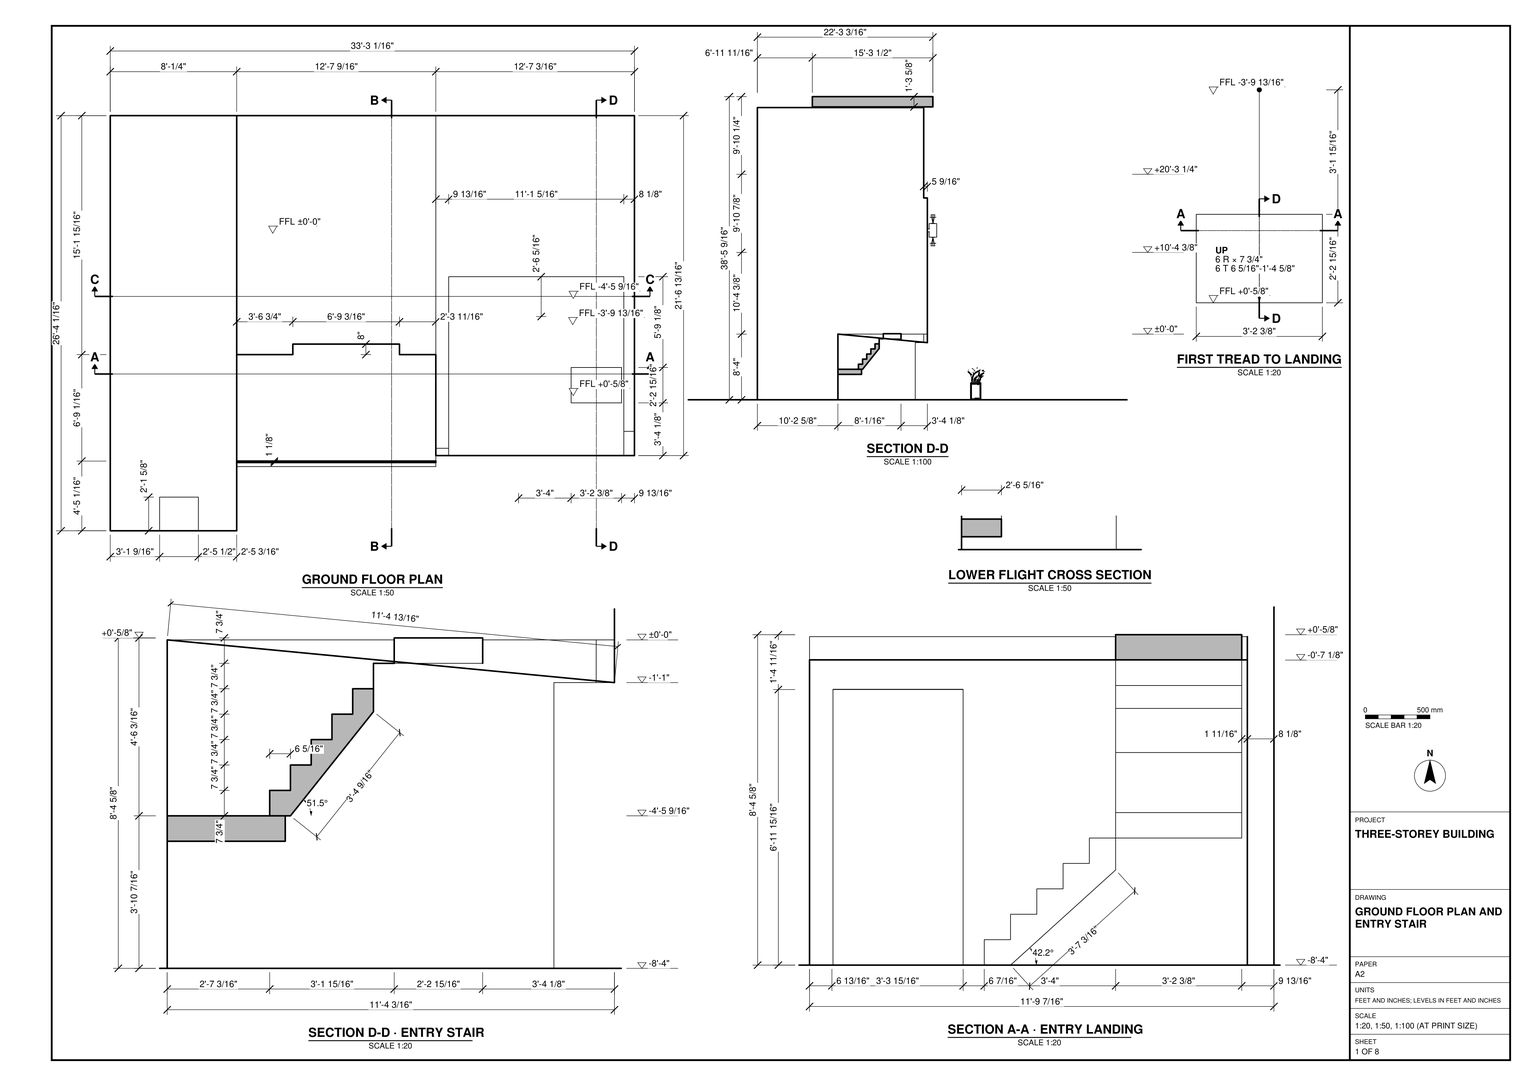
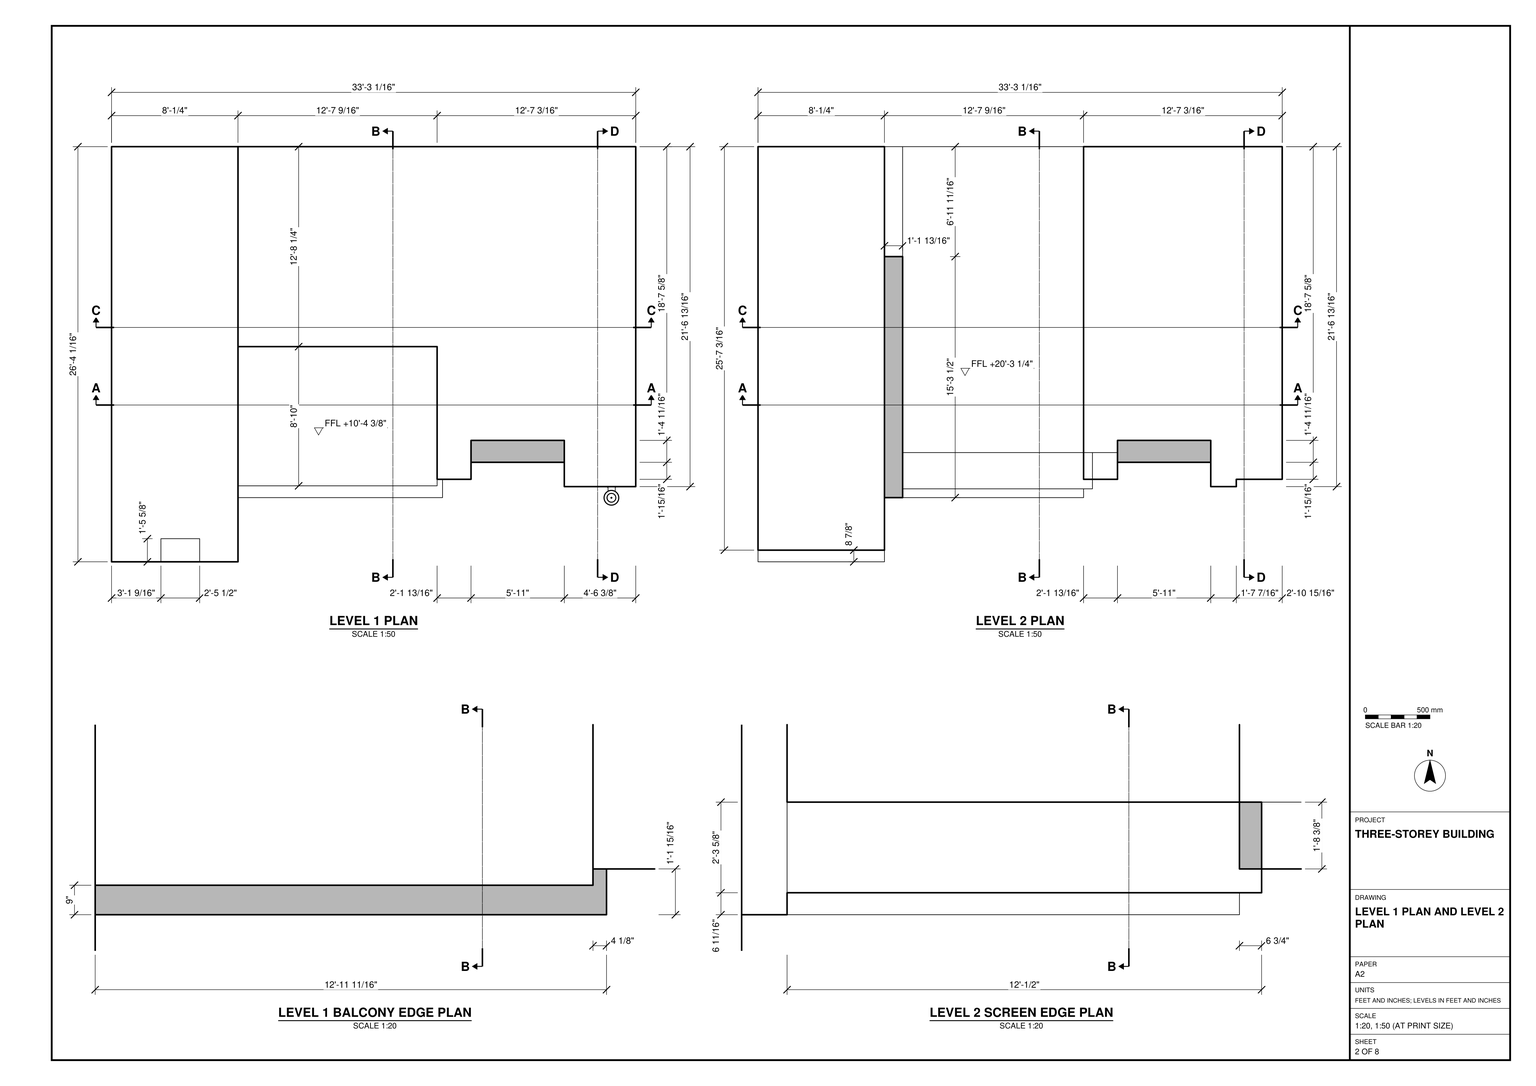
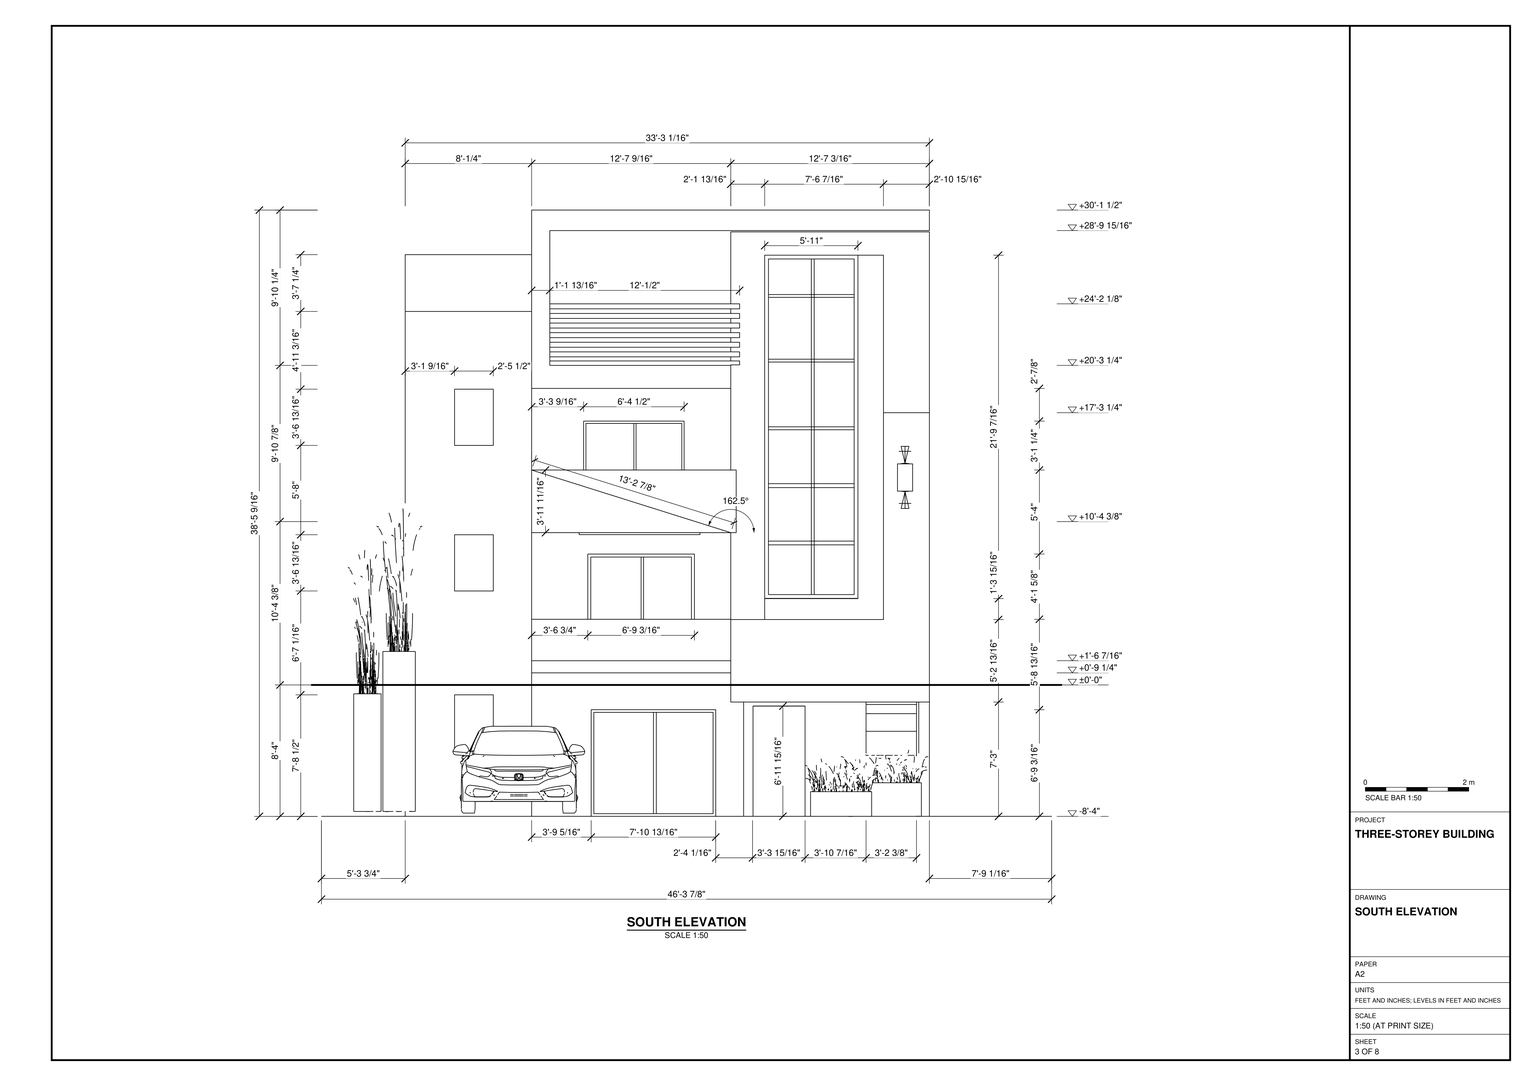
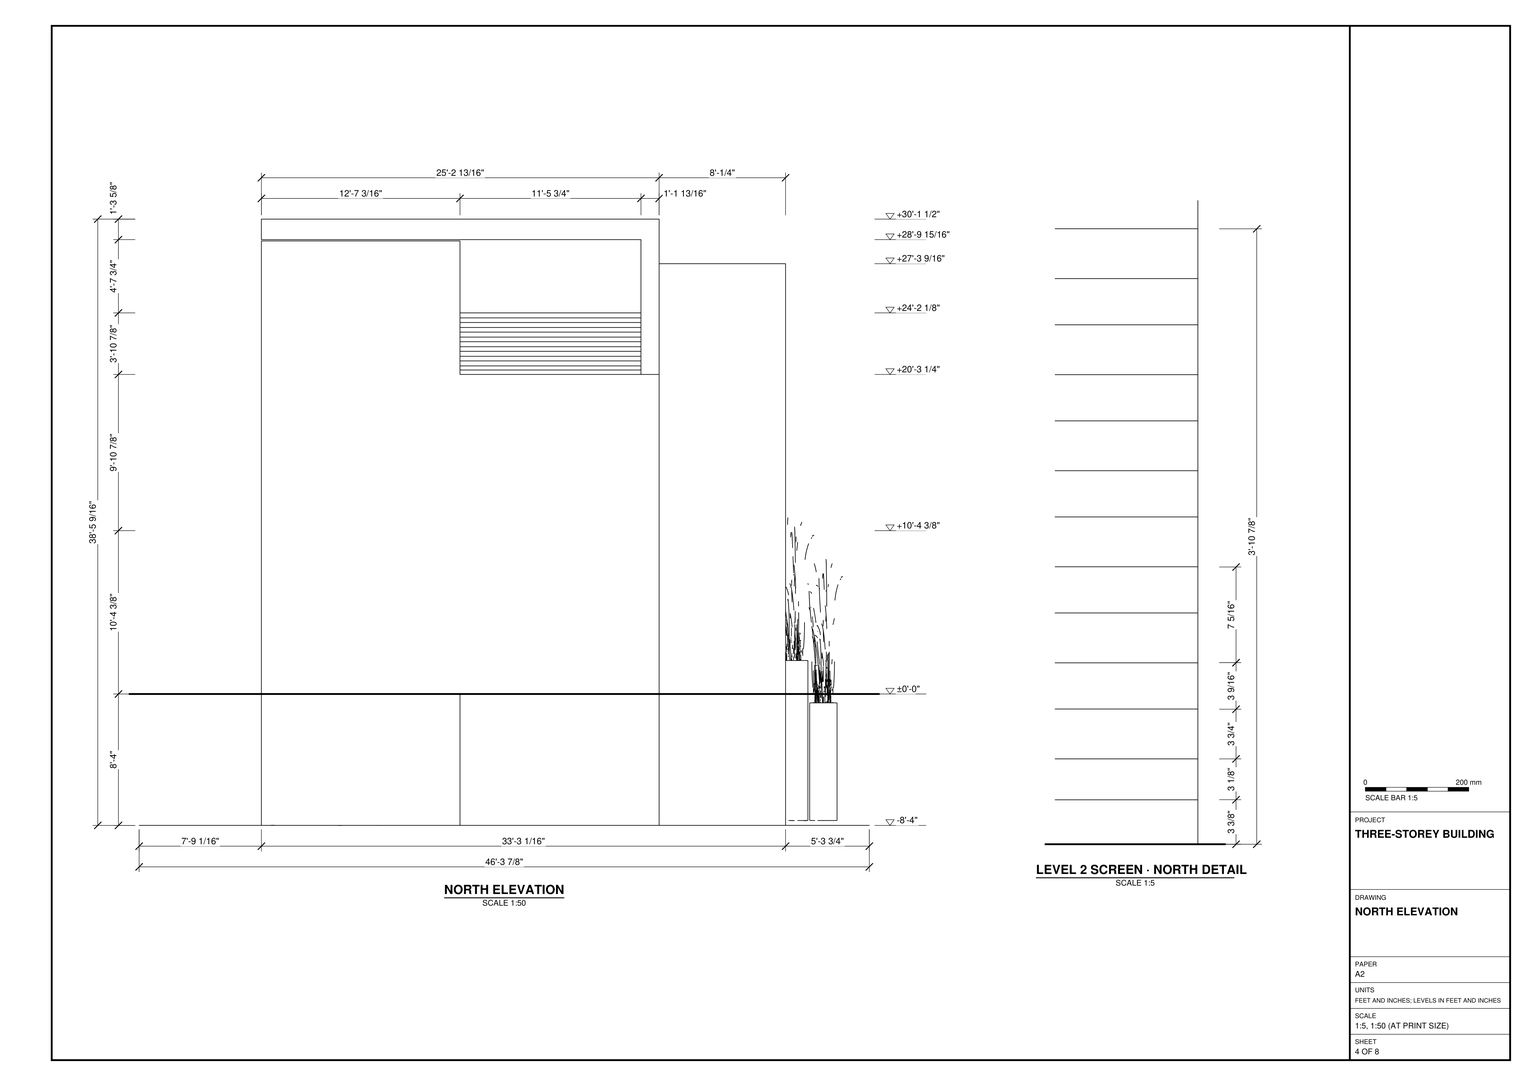
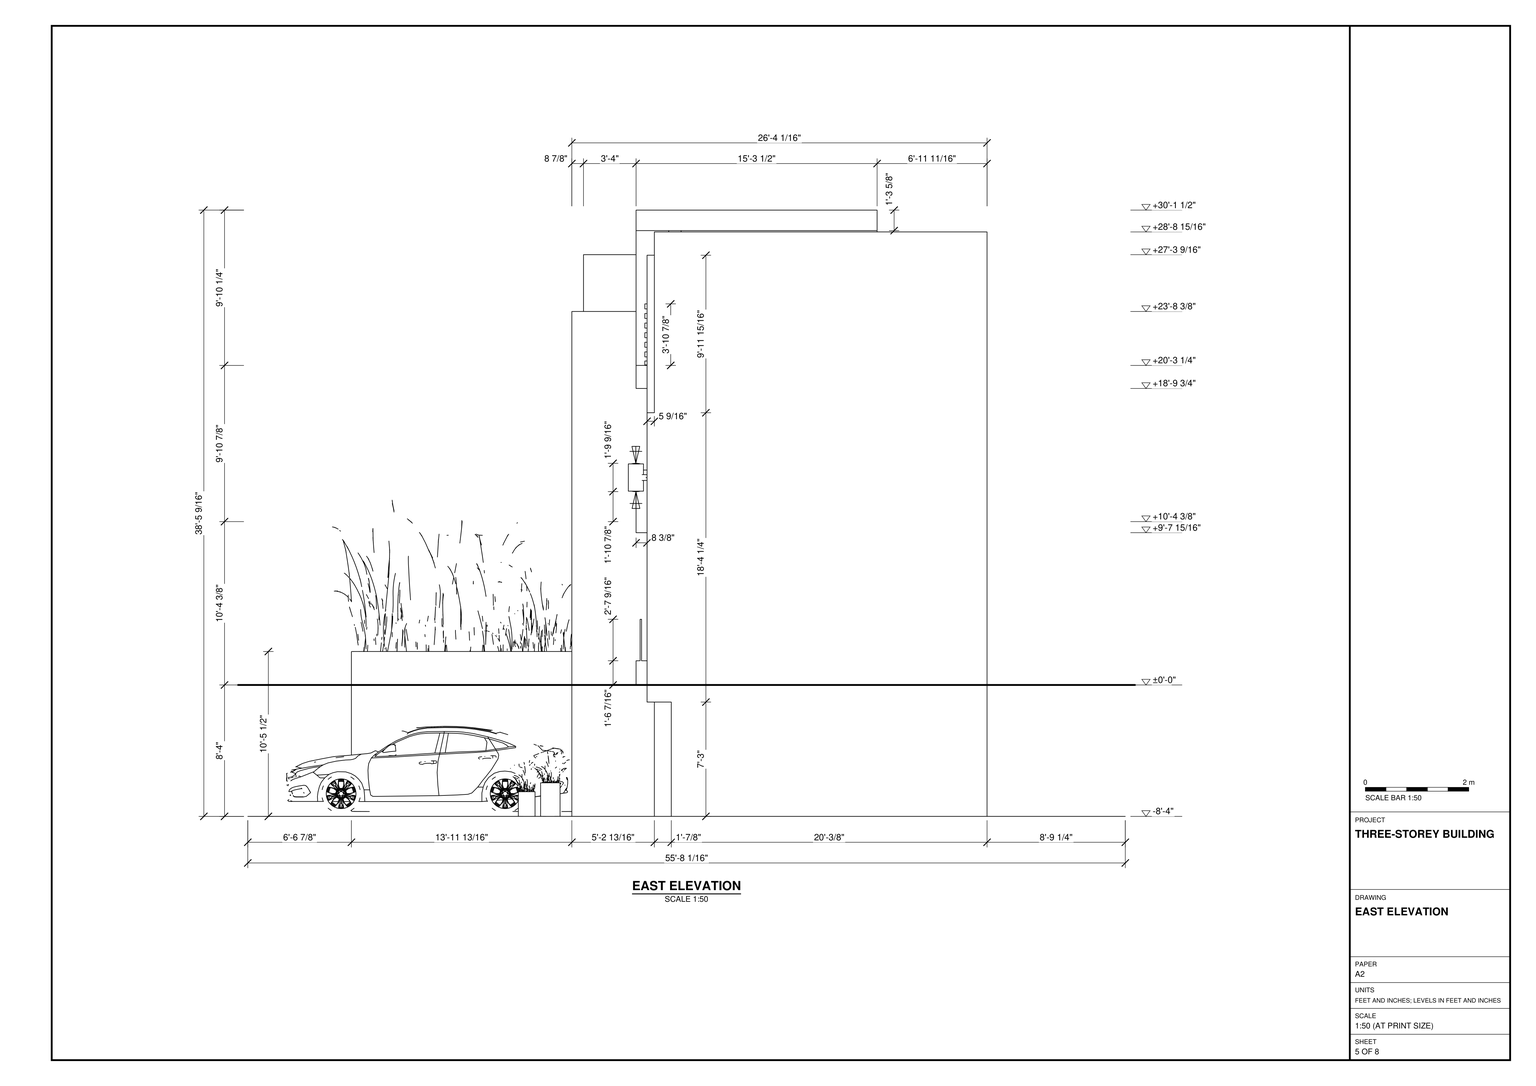
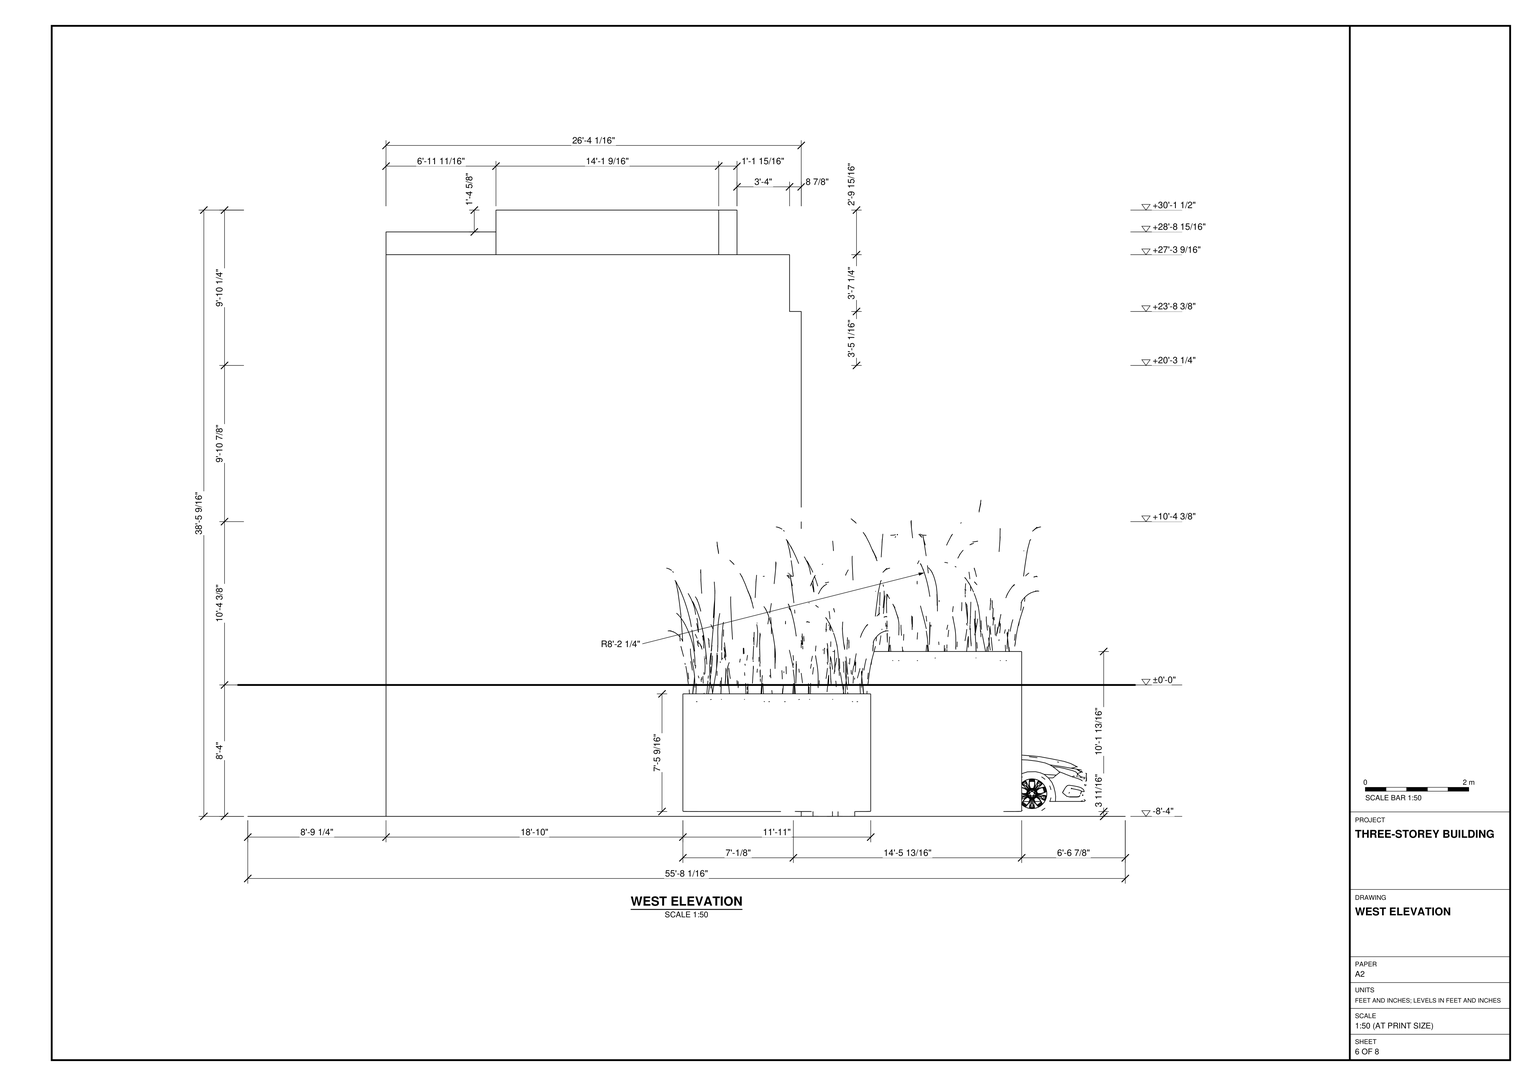
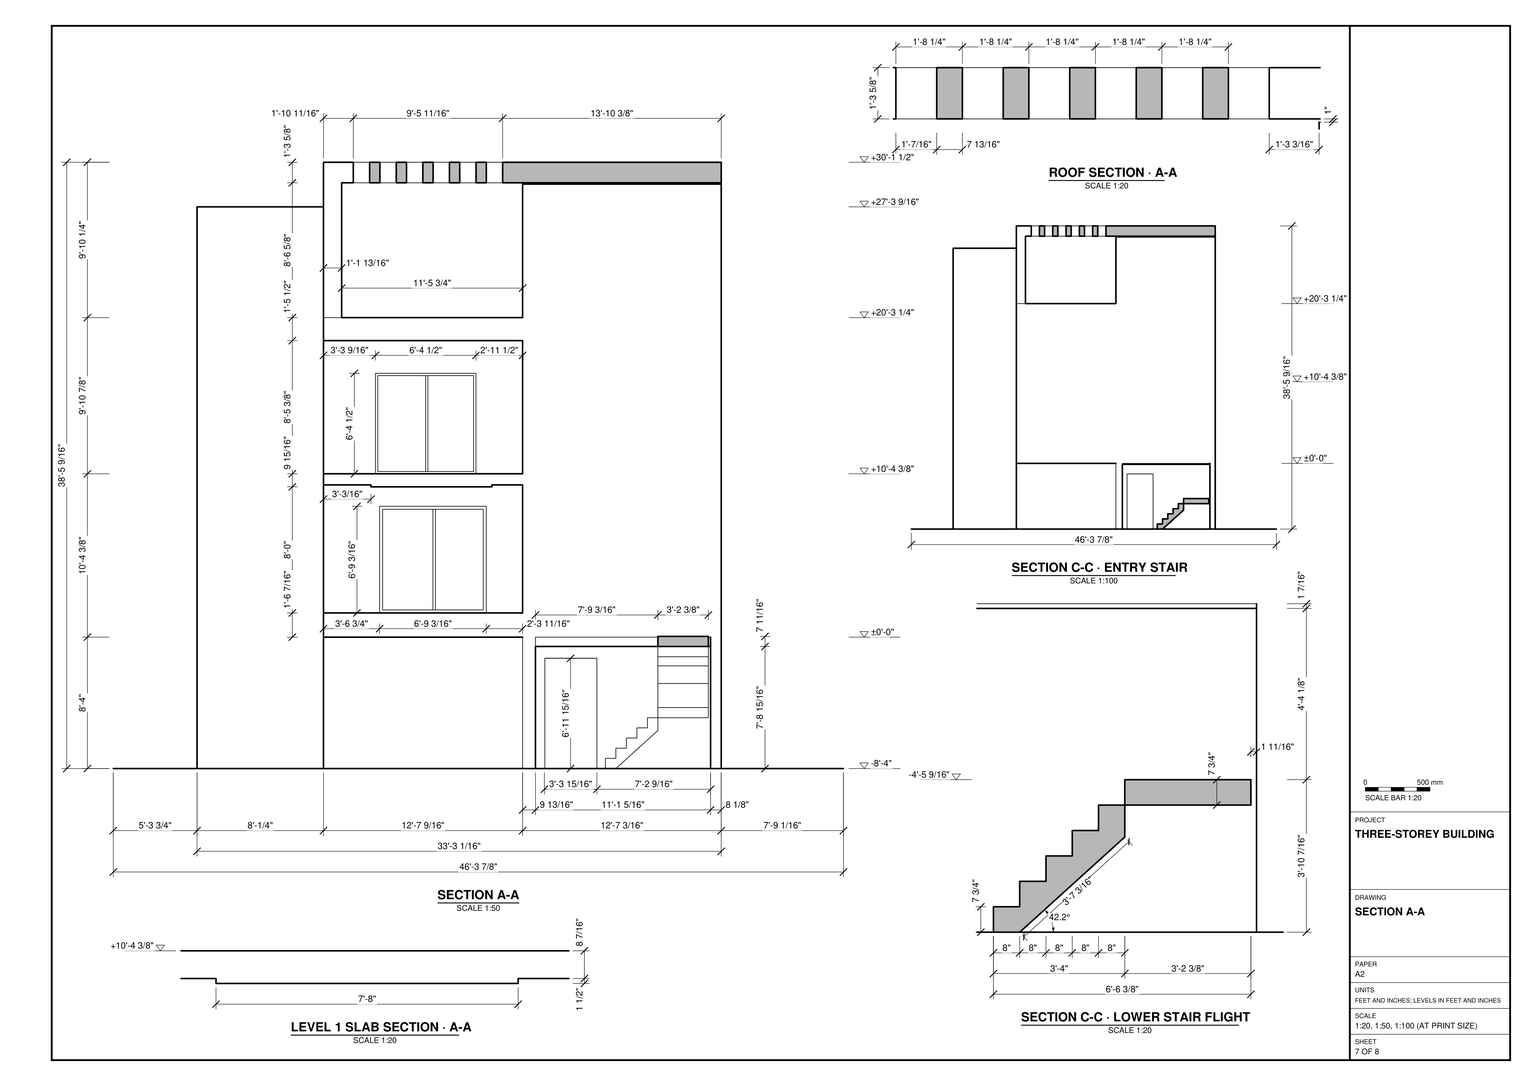
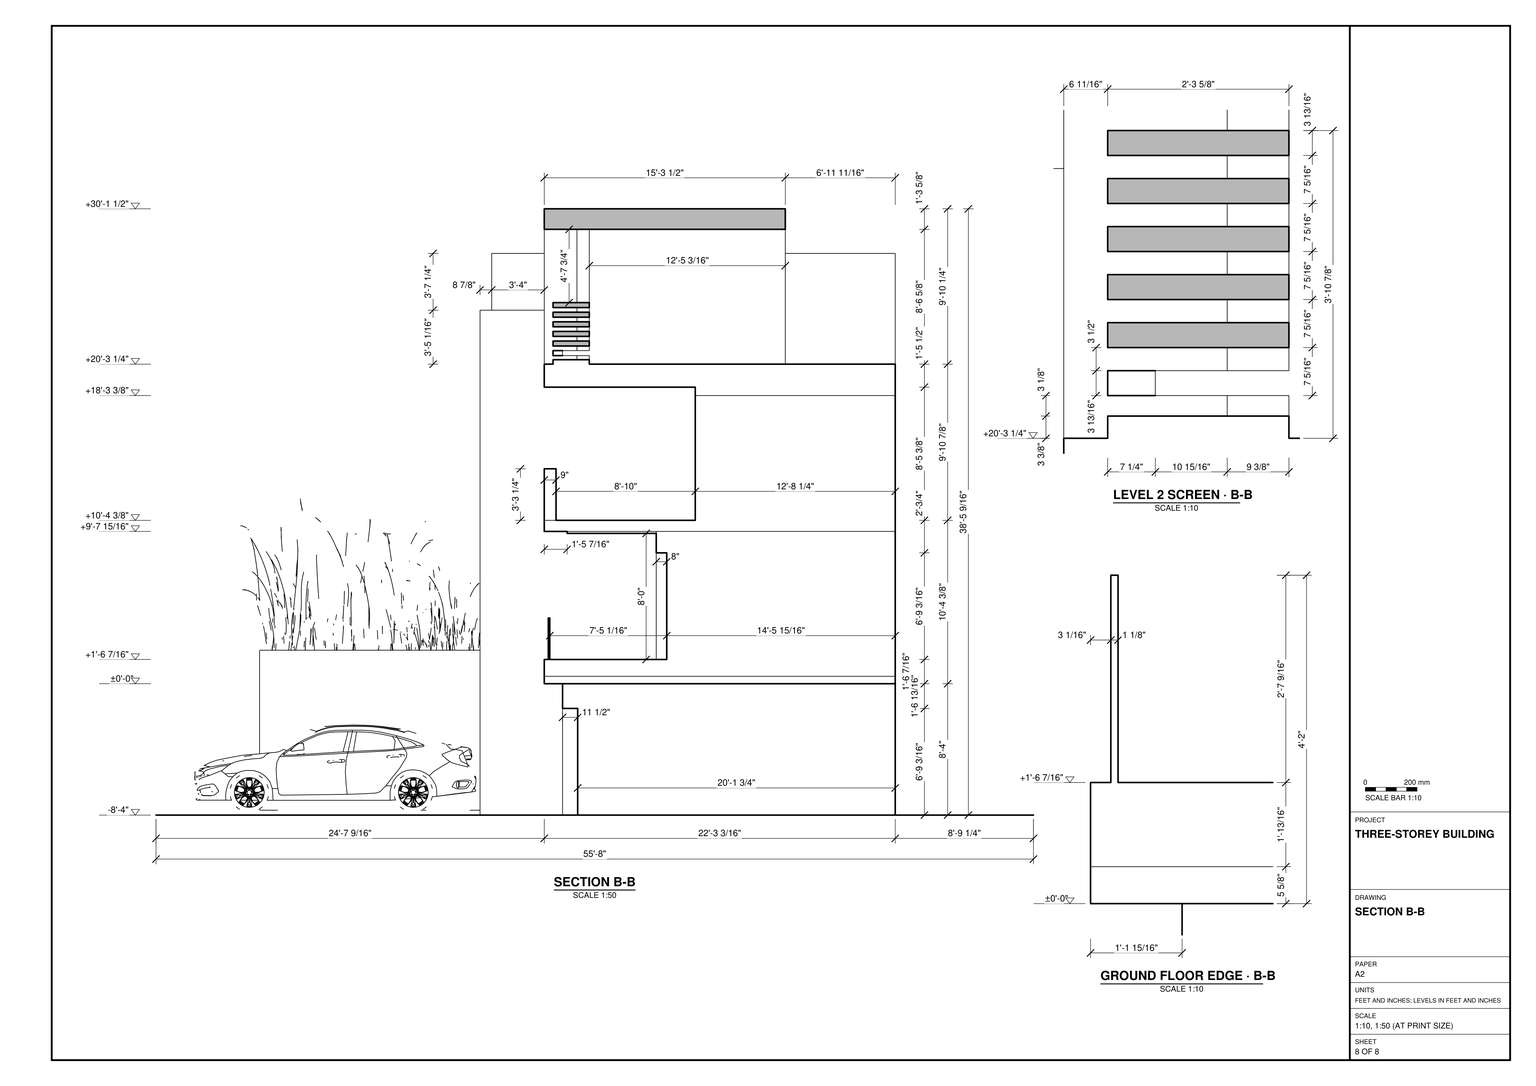
Build the three-storey building and its frontage in SketchUp from task_files/diagram_01.pdf. Work in feet and inches. The complete model, including the site, measures 46'-3 7/8" along X, 55'-8" along Y and 38'-5 9/16" along Z. Set the ground floor at ±0'-0", level 1 at +10'-4 3/8" and level 2 at +20'-3 1/4". The parking and entry approach are below the ground-floor datum.

Follow the stepped floor outlines in plan rather than stretching the building to the site boundaries. Model the walls at their drawn thicknesses, the floor slabs, door and window openings, and the flat roof with its changes in height. Use the entry sections to connect the lower approach to the raised entrance with stair flights and a turning landing.

On the south elevation, place the small stacked openings in the left wing, the projecting balcony and horizontal screen in the middle, and the tall framed glazing on the right. Match the slope of the balcony face and the divisions in the glazing. Include the parked car and frontage planters where shown. Decor and loose items may be any suitable library components. Keep walls, slabs, roof elements and each furniture or joinery piece shown in separate groups or components, and use components for repeated parts. Save one SketchUp model as output_files/three_storey_building_with_a_recessed_entry_stair.skp.

# SketchUp Ruby script. Lengths in inches.
U = 1.inch
M = Sketchup.active_model
def pt(a) = Geom::Point3d.new(a.map { |v| v * U })
def face(e, loops, mat)
  f = e.add_face(loops[0].map { |a| pt(a) })
  loops[1..].each { |l| e.add_face(l.map { |a| pt(a) }).erase! }
  f.material = f.back_material = mat if mat
  f
end
# faces: each face lists its corners as indices into pts; further lists are holes
def faces(e, pts, list, mat = nil) = list.each { |f| face(e, (f[0].is_a?(Array) ? f : [f]).map { |l| l.map { |i| pts[i] } }, mat) }
# xy, xz, yz: faces in a plane at the given z, y or x. An outline is a flat list of corners, or four numbers for a rectangle; further outlines are holes
def ring(l) = l.size == 4 ? [[l[0], l[1]], [l[2], l[1]], [l[2], l[3]], [l[0], l[3]]] : l.each_slice(2).to_a
def flat(e, list, mat, &to3) = list.each { |f| face(e, (f[0].is_a?(Array) ? f : [f]).map { |l| ring(l).map { |u, v| to3.(u, v) } }, mat) }
def xy(e, z, list, mat = nil) = flat(e, list, mat) { |x, y| [x, y, z] }
def xz(e, y, list, mat = nil) = flat(e, list, mat) { |x, z| [x, y, z] }
def yz(e, x, list, mat = nil) = flat(e, list, mat) { |y, z| [x, y, z] }
def lines(e, pts, list) = list.each { |a, b| e.add_line(pt(pts[a]), pt(pts[b])) }
# prism: a flat outline (further loops are holes) pulled along v
def prism(e, loops, v, mat = nil)
  f = face(e, loops, mat); d = Geom::Vector3d.new(v.map { |x| x * U })
  f.pushpull(f.normal.samedirection?(d) ? d.length : -d.length)
end
def box(e, o, s, mat = nil) = prism(e, [[o, [o[0] + s[0], o[1], o[2]], [o[0] + s[0], o[1] + s[1], o[2]], [o[0], o[1] + s[1], o[2]]]], [0, 0, s[2]], mat)
def at(x, y, z, deg = 0) = Geom::Transformation.translation(pt([x, y, z])) * Geom::Transformation.rotation(ORIGIN, Z_AXIS, deg.degrees)
def axes(o, x, y, z) = Geom::Transformation.new([*x, 0, *y, 0, *z, 0, *pt(o).to_a, 1])
def part(name) = M.definitions.add(name)
# library, detail: a bought-in or finely detailed component or shape, given as its bounding box
def library(name, o, s) = part(name).tap { |d| box(d.entities, o, s) }
def detail(e, o, s) = box(e.add_group.entities, o, s)
def put(e, d, t, mat = nil) = e.add_instance(d, t).tap { |i| i.material = mat if mat }
def group(e, t, mat = nil) = e.add_group.tap { |g| g.transformation = t; g.material = mat if mat }.entities
root = M.entities
M.materials.add("Niraj_Pant").color = [69, 86, 117]
M.materials.add("Niraj_Pant_Shadow").color = [70, 74, 99]
M.materials.add("[Asphalt New]").color = [67, 60, 62]
M.materials.add("[Concrete Form 4x8]").color = [167, 170, 168]
M.materials.add("[Translucent Glass Gray]").color = [128, 128, 128]
M.materials["[Translucent Glass Gray]"].alpha = 0.5
M.materials.add("[Wood Veneer 01]").color = [120, 70, 37]
c1 = part("steps")
xy(c1.entities,1.76,[[109.95,88,157.95,98]])
xy(c1.entities,9.26,[[109.95,88,157.95,98]])
xy(c1.entities,16.76,[[109.95,78,157.95,88]])
xy(c1.entities,24.26,[[109.95,68,157.95,78]])
xy(c1.entities,31.76,[[109.95,58,157.95,68]])
xy(c1.entities,39.26,[[101.08,0,157.95,48],[109.95,48,157.95,58]])
xy(c1.entities,46.76,[[98.58,0,101.08,48],[101.08,0,108.58,48],[108.58,0,157.95,48]])
xy(c1.entities,54.26,[[98.58,0,108.58,48]])
xy(c1.entities,61.76,[[88.58,0,98.58,48]])
xy(c1.entities,69.26,[[78.58,0,88.58,48]])
xy(c1.entities,76.76,[[68.58,0,78.58,48]])
xy(c1.entities,84.26,[[58.58,0,68.58,48]])
xy(c1.entities,91.76,[[48.58,0,58.58,48]])
xy(c1.entities,99.26,[[5.95,0,48.58,48]])
xz(c1.entities,0,[[101.08,39.26,157.95,46.76],[98.58,46.76,108.58,46.76,108.58,54.26,98.58,54.26,98.58,61.76,88.58,61.76,88.58,69.26,78.58,69.26,78.58,76.76,68.58,76.76,68.58,84.26,58.58,84.26,58.58,77.5,75.51,64.48],[5.95,91.76,48.58,99.26]])
xz(c1.entities,48,[[109.95,29.85,157.95,39.26],[101.08,39.26,157.95,46.76],[98.58,46.76,75.51,64.48,58.58,77.5,48.58,85.19,48.58,91.76,58.58,91.76,58.58,84.26,68.58,84.26,68.58,76.76,78.58,76.76,78.58,69.26,88.58,69.26,88.58,61.76,98.58,61.76,98.58,54.26,108.58,54.26,108.58,46.76],[5.95,91.76,48.58,99.26]])
xz(c1.entities,58,[[109.95,31.76,157.95,39.26]])
xz(c1.entities,68,[[109.95,24.26,157.95,31.76]])
xz(c1.entities,78,[[109.95,16.76,157.95,24.26]])
xz(c1.entities,88,[[109.95,9.26,157.95,16.76]])
xz(c1.entities,98,[[109.95,1.76,157.95,9.26]])
yz(c1.entities,5.95,[[0,91.76,48,99.26]])
yz(c1.entities,48.58,[[0,91.76,48,99.26]])
yz(c1.entities,58.58,[[0,84.26,48,91.76]])
yz(c1.entities,68.58,[[0,76.76,48,84.26]])
yz(c1.entities,78.58,[[0,69.26,48,76.76]])
yz(c1.entities,88.58,[[0,61.76,48,69.26]])
yz(c1.entities,98.58,[[0,54.26,48,61.76]])
yz(c1.entities,101.08,[[0,39.26,48,46.76]])
yz(c1.entities,108.58,[[0,46.76,48,54.26]])
yz(c1.entities,109.95,[[88,1.76,48,29.85,48,39.26,58,39.26,58,31.76,68,31.76,68,24.26,78,24.26,78,16.76,88,16.76,88,9.26,98,9.26,98,1.76]])
yz(c1.entities,157.95,[[88,1.76,98,1.76,98,9.26,88,9.26,88,16.76,78,16.76,78,24.26,68,24.26,68,31.76,58,31.76,58,39.26,48,39.26,48,29.85],[0,39.26,48,46.76]])
p = [[109.95,48,29.85],[109.95,88,1.76],[157.95,88,1.76],[157.95,48,29.85],[75.51,0,64.48],[75.51,48,64.48],
  [98.58,48,46.76],[98.58,0,46.76],[58.58,0,77.5],[58.58,48,77.5]]
faces(c1.entities,p,[[0,1,2,3],[4,5,6,7],[8,9,5,4]])
c2 = part("DOOR12")
g1 = group(c2.entities,at(114.73,28.14,-0.51))
g2 = group(g1,at(0,0,0))
box(g2,[0,0,0],[36,0.5,77.7])
c3 = library("House+plant_11",[9.78,20.5,0],[94.8,46.14,50.64])
c4 = library("car\#1",[0.01,0.03,0.02],[18.76,39.97,12.32])
c5 = library("WALL+LIGHT+69",[4.19,4.05,-9.67],[4.61,5.7,18.91])
xy(root,0,[[[0,0,555.875,668],[63.77,203.32,462.58,203.32,462.58,322.38,462.8125,322.38,462.8125,562.76,63.77,562.76]],[63.77,246.7,160.03,562.76],[160.03,309.51,160.03,562.76,311.61,562.76,311.61,309.51,300.16,309.51,300.16,321.01,205.35,321.01,205.35,309.51],[311.61,309.51,311.61,562.76,462.58,562.76,462.58,440.13,368.17,440.13,368.17,467.95,328.54,467.95,328.54,440.13,321.4,440.13,321.4,309.51],[321.4,309.51,321.4,440.13,328.54,440.13,328.54,467.95,368.17,467.95,368.17,440.13,454.71,440.13,454.71,309.51],
  [454.71,322.38,462.58,440.13],[462.58,322.38,462.8125,440.13],[462.58,440.13,462.8125,562.76]])
xy(root,0,[[63.77,203.32,63.77,246.7,160.03,246.7,160.03,309.51,205.35,309.51,205.35,321.01,300.16,321.01,300.16,309.51,454.71,309.51,454.71,322.38,462.58,322.38,462.58,203.32]],"[Concrete Form 4x8]")
xy(root,49.69,[[101.34,246.7,130.84,272.32]])
xy(root,81.1875,[[205.35,309.51,300.16,321.01]])
xy(root,84,[[328.54,440.13,368.17,467.95]])
xy(root,87.02,[[311.61,303.95,321.4,309.51],[454.71,303.95,462.8125,322.38]])
xy(root,92.51,[[101.34,246.7,130.84,272.32]])
xy(root,100.02,[[160.03,295.57,311.61,309.51],[160.03,309.51,311.61,562.76]])
xy(root,118.47,[[160.03,295.57,311.61,298.66],[160.03,299.76,311.61,299.76,311.61,380.82,283.95,380.82,283.95,388.82,202.76,388.82,202.76,380.82,160.03,380.82]])
xy(root,149.83,[[311.61,303.95,337.42,309.51]])
xy(root,150.03,[[160.03,298.66,311.61,299.76]])
xy(root,165.74,[[337.42,303.95,408.42,309.51]])
xy(root,165.93,[[337.42,309.51,408.42,322.45],[337.42,322.45,408.42,339.13]])
xy(root,171.57,[[101.34,246.7,130.84,264.32]])
xy(root,199.65,[[202.76,380.82,283.95,388.82]])
xy(root,214.38,[[101.34,246.7,130.84,264.32]])
xy(root,214.46,[[196.18,313.01,288.18,380.82]])
xy(root,215.96,[[160.03,295.57,160.03,380.82,196.18,380.82,196.18,313.01,288.18,313.01,288.18,380.82,311.61,380.82,311.61,309.51,315.73,309.51,315.73,295.57]])
xy(root,224.4,[[160.03,304.54,311.61,410.53]])
xy(root,263.65,[[160.03,295.57,315.73,295.57,315.73,309.51,311.61,309.51,311.61,304.54,160.03,304.54]])
xy(root,282.38,[[101.34,246.7,130.84,273.07]])
xy(root,307.29,[[427.86,303.95,462.8125,309.51]])
xy(root,325.19,[[101.34,246.7,130.84,273.07]])
xy(root,325.77,[[160.03,295.57,311.61,410.53]])
xy(root,343.3,[[173.86,295.57,311.61,302.26],[173.86,329.85,311.61,562.76],[160.03,479.07,173.86,562.76]])
xy(root,343.71,[[311.61,302.26,318.36,309.51]])
xy(root,346.6875,[[173.86,302.26,318.36,302.26,318.36,309.51,311.61,309.51,311.61,329.85,173.86,329.85]])
xy(root,349.8,[[173.86,302.26,311.61,309.51],[311.61,302.26,318.36,309.51]])
xy(root,353.6,[[173.86,302.26,318.36,309.51]])
xy(root,357.12,[[173.86,302.26,318.36,329.85]],"[Wood Veneer 01]")
xy(root,360.91,[[173.86,302.26,318.36,329.85]])
xy(root,364.43,[[173.86,302.26,318.36,329.85]],"[Wood Veneer 01]")
xy(root,368.22,[[173.86,302.26,318.36,329.85]])
xy(root,371.74,[[173.86,302.26,318.36,329.85]],"[Wood Veneer 01]")
xy(root,375.54,[[173.86,302.26,318.36,329.85]])
xy(root,379.05,[[173.86,302.26,318.36,329.85]],"[Wood Veneer 01]")
xy(root,382.85,[[173.86,302.26,318.36,329.85]])
xy(root,384.38,[[63.77,246.7,160.03,255.57]])
xy(root,386.37,[[173.86,302.26,318.36,329.85]],"[Wood Veneer 01]")
xy(root,390.16,[[173.86,302.26,318.36,329.85]])
xy(root,427.2,[[408.42,303.95,427.86,309.51],[337.42,309.51,408.42,322.45],[337.42,322.45,408.42,339.13]])
xy(root,427.62,[[63.77,255.57,160.03,562.76]])
xy(root,444.9375,[[311.61,309.51,462.8125,562.76]])
xy(root,445.94,[[[173.86,295.57,462.8125,479.07],[182.73,350.06,195.17,443.93],[202.98,350.06,215.42,443.93],[223.23,350.06,235.67,443.93],[243.48,350.06,255.92,443.93],[263.73,350.06,276.17,443.93],[283.98,350.06,296.42,443.93]]])
xy(root,461.55,[[[160.03,295.57,462.8125,479.07],[182.73,350.06,195.17,443.93],[202.98,350.06,215.42,443.93],[223.23,350.06,235.67,443.93],[243.48,350.06,255.92,443.93],[263.73,350.06,276.17,443.93],[283.98,350.06,296.42,443.93]]])
xz(root,246.7,[[[63.77,0,160.03,384.38],[101.34,282.38,130.84,325.19],[101.34,171.57,130.84,214.38],[101.34,49.69,130.84,92.51]]])
xz(root,255.57,[[63.77,384.38,160.03,427.62]],"Niraj_Pant")
xz(root,264.32,[[101.34,171.57,130.84,214.38]],"[Translucent Glass Gray]")
xz(root,272.32,[[101.34,49.69,130.84,92.51]],"[Translucent Glass Gray]")
xz(root,273.07,[[101.34,282.38,130.84,325.19]],"[Translucent Glass Gray]")
xz(root,295.57,[[160.03,100.02,311.61,109.25],[160.03,215.96,311.61,215.96,160.03,263.65],[311.61,215.96,315.73,215.96,315.73,263.65,160.03,263.65],[160.03,325.77,311.61,325.77,311.61,343.3,173.86,343.3,173.86,445.94,462.8125,445.94,462.8125,461.55,160.03,461.55]])
xz(root,295.57,[[160.03,109.25,311.61,118.47]],"Niraj_Pant_Shadow")
xz(root,298.66,[[160.03,118.47,311.61,150.03]],"[Translucent Glass Gray]")
xz(root,299.76,[[160.03,118.47,311.61,150.03]],"[Translucent Glass Gray]")
xz(root,302.26,[[173.86,343.3,311.61,343.3,311.61,343.71,318.36,343.71,318.36,346.6875,173.86,346.6875],[173.86,349.8,318.36,353.6],[173.86,357.12,318.36,360.91],[173.86,364.43,318.36,368.22],[173.86,371.74,318.36,375.54],
  [173.86,379.05,318.36,382.85],[173.86,386.37,318.36,390.16]],"[Wood Veneer 01]")
xz(root,303.95,[[311.61,87.02,462.8125,87.02,462.8125,307.29,427.86,307.29,427.86,149.83,311.61,149.83],[337.42,149.83,427.86,149.83,427.86,427.2,408.42,427.2,408.42,165.74,337.42,165.74]])
xz(root,304.54,[[160.03,224.4,311.61,263.65]])
xz(root,309.51,[[160.03,0,205.35,0,205.35,81.1875,300.16,81.1875,300.16,0,321.4,0,321.4,87.02,311.61,87.02,311.61,100.02,160.03,100.02],[337.42,165.74,408.42,165.93],[311.61,224.4,315.73,263.65],[311.61,343.71,318.36,346.6875],[311.61,349.8,318.36,353.6]])
xz(root,309.51,[[311.61,149.83,337.42,149.83,337.42,427.2,427.86,427.2,427.86,307.29,462.8125,307.29,462.8125,444.9375,311.61,444.9375,311.61,353.6,318.36,353.6,318.36,349.8,311.61,349.8,311.61,346.6875,318.36,346.6875,318.36,343.71,311.61,343.71,311.61,263.65,315.73,263.65,315.73,215.96,311.61,215.96]],"Niraj_Pant")
xz(root,313.01,[[196.18,214.46,288.18,215.96]])
xz(root,321.01,[[[205.35,0,300.16,81.1875],[207.36,2.02,298.14,79.17]],[252.75,2.02,254.9375,79.17]],"[Asphalt New]")
xz(root,321.01,[[207.36,2.02,252.75,79.17],[254.9375,2.02,298.14,79.17]],"[Translucent Glass Gray]")
xz(root,322.38,[[454.71,0,462.8125,87.02]])
xz(root,322.45,[[[337.42,165.93,408.42,427.2],[340.31,168.82,405.53,424.32]],[372.92,168.82,375.11,206.69],[340.31,206.69,372.92,209.54],[372.92,206.69,375.11,209.54],[375.11,206.69,405.53,209.54],
  [372.92,209.54,375.11,250.27],[340.31,250.27,372.92,253.26],[372.92,250.27,375.11,253.26],[375.11,250.27,405.53,253.26],[372.92,253.26,375.11,294.31],
  [340.31,294.31,372.92,296.57],[372.92,294.31,375.11,296.57],[375.11,294.31,405.53,296.57],[372.92,296.57,375.11,345.84],[340.31,345.84,372.92,348.02],
  [372.92,345.84,375.11,348.02],[375.11,345.84,405.53,348.02],[372.92,348.02,375.11,395.12],[340.31,395.12,372.92,397.24],[372.92,395.12,375.11,397.24],
  [375.11,395.12,405.53,397.24],[372.92,397.24,375.11,424.32]],"[Asphalt New]")
xz(root,322.45,[[340.31,168.82,372.92,206.69],[375.11,168.82,405.53,206.69],[340.31,209.54,372.92,250.27],[375.11,209.54,405.53,250.27],[340.31,253.26,372.92,294.31],
  [375.11,253.26,405.53,294.31],[340.31,296.57,372.92,345.84],[375.11,296.57,405.53,345.84],[340.31,348.02,372.92,395.12],[375.11,348.02,405.53,395.12],
  [340.31,397.24,372.92,424.32],[375.11,397.24,405.53,424.32]],"[Translucent Glass Gray]")
xz(root,329.85,[[173.86,343.3,311.61,346.6875],[173.86,357.12,318.36,360.91],[173.86,364.43,318.36,368.22],[173.86,371.74,318.36,375.54],[173.86,379.05,318.36,382.85],
  [173.86,386.37,318.36,390.16]])
xz(root,339.13,[[337.42,165.93,408.42,427.2]])
xz(root,350.06,[[182.73,445.94,195.17,461.55],[202.98,445.94,215.42,461.55],[223.23,445.94,235.67,461.55],[243.48,445.94,255.92,461.55],[263.73,445.94,276.17,461.55],
  [283.98,445.94,296.42,461.55]])
xz(root,377.33,[[414.6,78.17,453,85.14],[414.6,85.14,453,92.88]])
xz(root,380.82,[[160.03,118.47,202.76,118.47,202.76,199.65,283.95,199.65,283.95,118.47,311.61,118.47,311.61,215.96,288.18,215.96,288.18,214.46,196.18,214.46,196.18,215.96,160.03,215.96]])
xz(root,388.82,[[[202.76,118.47,283.95,199.65],[205.03,120.74,281.67,197.38]],[243.35,120.74,245.24,197.38]],"[Asphalt New]")
xz(root,388.82,[[205.03,120.74,243.35,197.38],[245.24,120.74,281.67,197.38]],"[Translucent Glass Gray]")
xz(root,410.53,[[160.03,224.4,199.6,224.4,199.6,300.9,276.1,300.9,276.1,224.4,311.61,224.4,311.61,325.77,160.03,325.77]])
xz(root,410.53,[[[199.6,224.4,276.1,300.9],[201.35,226.15,274.35,299.15]],[237.85,226.15,239.5,299.15]],"[Asphalt New]")
xz(root,410.53,[[201.35,226.15,237.85,299.15],[239.5,226.15,274.35,299.15]],"[Translucent Glass Gray]")
xz(root,440.13,[[321.4,0,328.54,0,328.54,84,368.17,84,368.17,0,454.71,0,454.71,100.02,321.4,100.02]])
xz(root,443.93,[[182.73,445.94,195.17,461.55],[202.98,445.94,215.42,461.55],[223.23,445.94,235.67,461.55],[243.48,445.94,255.92,461.55],[263.73,445.94,276.17,461.55],
  [283.98,445.94,296.42,461.55]])
xz(root,467.95,[[328.54,0,368.17,84]])
xz(root,479.07,[[160.03,343.3,160.03,461.55,462.8125,461.55,462.8125,445.94,173.86,445.94,173.86,343.3]])
xz(root,562.76,[[63.77,0,160.03,427.62],[160.03,0,311.61,100.02],[311.61,0,311.61,100.02,160.03,100.02,160.03,343.3,311.61,343.3,311.61,444.9375,462.8125,444.9375,462.8125,0]])
yz(root,63.77,[[246.7,0,246.7,384.38,255.57,384.38,255.57,427.62,562.76,427.62,562.76,0]])
yz(root,101.34,[[246.7,49.69,272.32,92.51],[246.7,171.57,264.32,214.38],[246.7,282.38,273.07,325.19]])
yz(root,130.84,[[246.7,49.69,272.32,92.51],[246.7,171.57,264.32,214.38],[246.7,282.38,273.07,325.19]])
yz(root,160.03,[[246.7,0,309.51,0,309.51,100.02,295.57,100.02,295.57,118.47,298.66,118.47,298.66,150.03,299.76,150.03,299.76,118.47,380.82,118.47,380.82,215.96,295.57,215.96,295.57,263.65,304.54,263.65,304.54,224.4,410.53,224.4,410.53,325.77,295.57,325.77,295.57,384.38,246.7,384.38],[309.51,0,562.76,100.02],[295.57,100.02,562.76,105.65],[295.57,105.65,295.57,118.47,298.66,118.47,298.66,150.03,299.76,150.03,299.76,118.47,380.82,118.47,380.82,215.96,562.76,215.96,562.76,105.65],[295.57,215.96,562.76,215.96,562.76,319.4,410.53,319.4,410.53,224.4,295.57,224.4],
  [295.57,224.4,304.54,263.65],[410.53,319.4,562.76,319.4,562.76,343.3,479.07,343.3,479.07,427.62,295.57,427.62,295.57,325.77,410.53,325.77],[479.07,343.3,562.76,427.62],[295.57,427.62,309.51,461.55],[309.51,427.62,479.07,461.55]])
yz(root,160.03,[[255.57,384.38,295.57,427.62]],"Niraj_Pant")
yz(root,173.86,[[295.57,343.3,302.26,343.3,302.26,346.6875,320.45,346.6875,320.45,349.8,309.51,349.8,309.51,353.6,320.45,353.6,320.45,357.12,302.26,357.12,302.26,360.91,320.45,360.91,320.45,364.43,302.26,364.43,302.26,368.22,320.45,368.22,320.45,371.74,302.26,371.74,302.26,375.54,320.45,375.54,320.45,379.05,302.26,379.05,302.26,382.85,320.45,382.85,320.45,386.37,302.26,386.37,302.26,390.16,320.45,390.16,320.45,445.94,295.57,445.94],[329.85,343.3,479.07,343.3,479.07,445.94,329.85,445.94,329.85,353.6,309.51,353.6,309.51,349.8,329.85,349.8],[320.45,346.6875,329.85,349.8],[320.45,353.6,329.85,357.12],[320.45,360.91,329.85,364.43],
  [320.45,368.22,329.85,371.74],[320.45,375.54,329.85,379.05],[320.45,382.85,329.85,386.37],[320.45,390.16,329.85,445.94]])
yz(root,182.73,[[350.06,445.94,443.93,461.55]])
yz(root,195.17,[[350.06,445.94,443.93,461.55]])
yz(root,196.18,[[313.01,214.46,380.82,215.96]])
yz(root,202.76,[[380.82,118.47,388.82,199.65]])
yz(root,202.98,[[350.06,445.94,443.93,461.55]])
yz(root,205.35,[[309.51,0,321.01,81.1875]])
yz(root,215.42,[[350.06,445.94,443.93,461.55]])
yz(root,223.23,[[350.06,445.94,443.93,461.55]])
yz(root,235.67,[[350.06,445.94,443.93,461.55]])
yz(root,243.48,[[350.06,445.94,443.93,461.55]])
yz(root,255.92,[[350.06,445.94,443.93,461.55]])
yz(root,263.73,[[350.06,445.94,443.93,461.55]])
yz(root,276.17,[[350.06,445.94,443.93,461.55]])
yz(root,283.95,[[380.82,118.47,388.82,199.65]])
yz(root,283.98,[[350.06,445.94,443.93,461.55]])
yz(root,288.18,[[313.01,214.46,380.82,215.96]])
yz(root,296.42,[[350.06,445.94,443.93,461.55]])
yz(root,300.16,[[309.51,0,321.01,81.1875]])
yz(root,311.61,[[303.95,87.02,309.51,100.02],[295.57,100.02,303.95,100.02,303.95,118.47,299.76,118.47,299.76,150.03,298.66,150.03,298.66,118.47,295.57,118.47],[303.95,118.47,303.95,149.83,309.51,149.83,309.51,215.96,380.82,215.96,380.82,118.47],[304.54,224.4,309.51,263.65],[309.51,224.4,410.53,325.77],
  [295.57,325.77,309.51,343.3],[302.26,343.3,309.51,343.71],[309.51,343.3,329.85,346.6875],[329.85,343.3,562.76,343.3,562.76,444.9375,309.51,444.9375,309.51,346.6875,329.85,346.6875]])
yz(root,315.73,[[295.57,215.96,309.51,263.65]])
yz(root,318.36,[[302.26,343.71,309.51,346.6875],[302.26,349.8,309.51,353.6],[302.26,357.12,329.85,360.91],[302.26,364.43,329.85,368.22],[302.26,371.74,329.85,375.54],
  [302.26,379.05,329.85,382.85],[302.26,386.37,329.85,390.16]])
yz(root,321.4,[[309.51,0,440.13,0,440.13,100.02,303.95,87.02,309.51,87.02]])
yz(root,328.54,[[440.13,0,467.95,84]])
yz(root,337.42,[[303.95,149.83,309.51,165.74],[309.51,165.93,322.45,427.2],[322.45,165.93,339.13,427.2]])
yz(root,368.17,[[440.13,0,467.95,84]])
yz(root,408.42,[[303.95,165.74,303.95,427.2,322.45,427.2,322.45,165.93,309.51,165.93,309.51,165.74],[322.45,165.93,339.13,427.2]])
yz(root,427.86,[[303.95,307.29,309.51,427.2]])
yz(root,454.71,[[322.38,0,322.38,87.02,309.51,87.02,309.51,87.55,440.13,100.02,440.13,0],[303.95,87.02,309.51,87.55,309.51,87.02],[309.51,87.55,309.51,100.02,440.13,100.02]])
yz(root,462.8125,[[322.38,0,562.76,0,562.76,444.9375,309.51,444.9375,309.51,307.29,303.95,307.29,303.95,87.02,322.38,87.02],[295.57,445.94,479.07,461.55]])
p = [[321.4,303.95,87.02],[321.4,440.13,100.02],[454.71,440.13,100.02],[454.71,309.51,87.55],[454.71,303.95,87.02],[321.4,303.95,100.02],
  [454.71,303.95,100.02],[454.71,309.51,100.02],[337.42,329.85,349.8],[337.42,322.45,349.8],[173.86,329.85,353.6],[337.42,329.85,353.6],
  [173.86,329.85,349.8],[337.42,322.45,353.6]]
faces(root,p,[[0,1,2,3,4]])
lines(root,p,[[5,1],[6,7],[8,9],[10,11],[12,8],[13,11]])
put(root,c1,axes([453,340.31,-1.8125],[0,0.632,0],[-0.8,0,0],[0,0,1.032]))
put(root,c2,axes([200.86,579.53,0.55],[1.11,0,0],[0,-4.85,0],[0,0,1.08]))
put(root,c3,at(357.75,178.84,0))
put(root,c3,axes([-5.51,379.16,3.71],[0.18733,-3.06288,0],[0.99813,0.06105,0],[0,0,4.7664]))
put(root,c4,axes([99.88,28.79,2.35],[5.3692,0,0],[0,5.3692,0],[0,0,5.3692]))
put(root,c5,axes([428.04,279.58,258.58],[2.5,0,0],[0,2.5,0],[0,0,2.5]))
